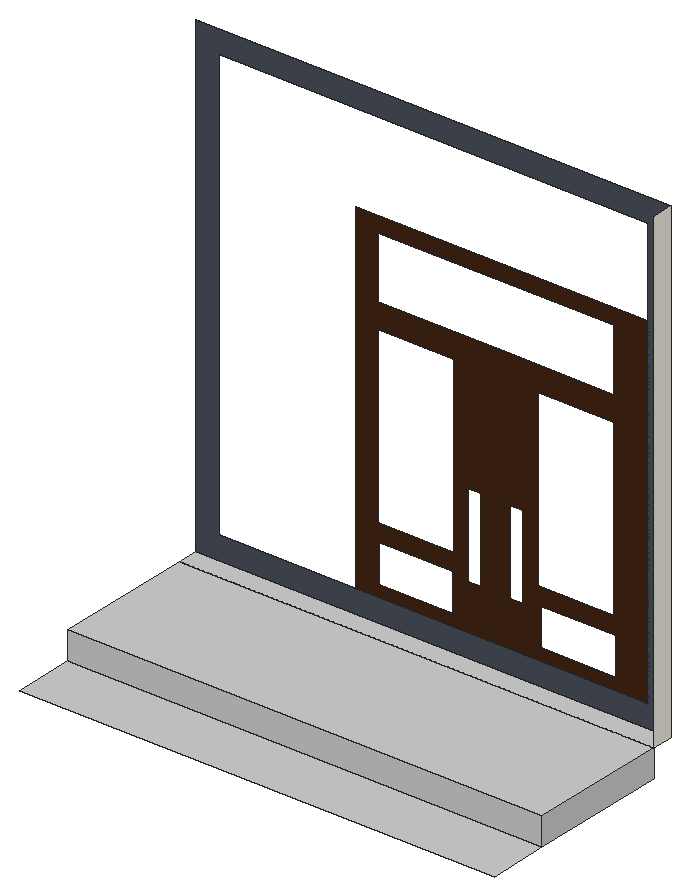
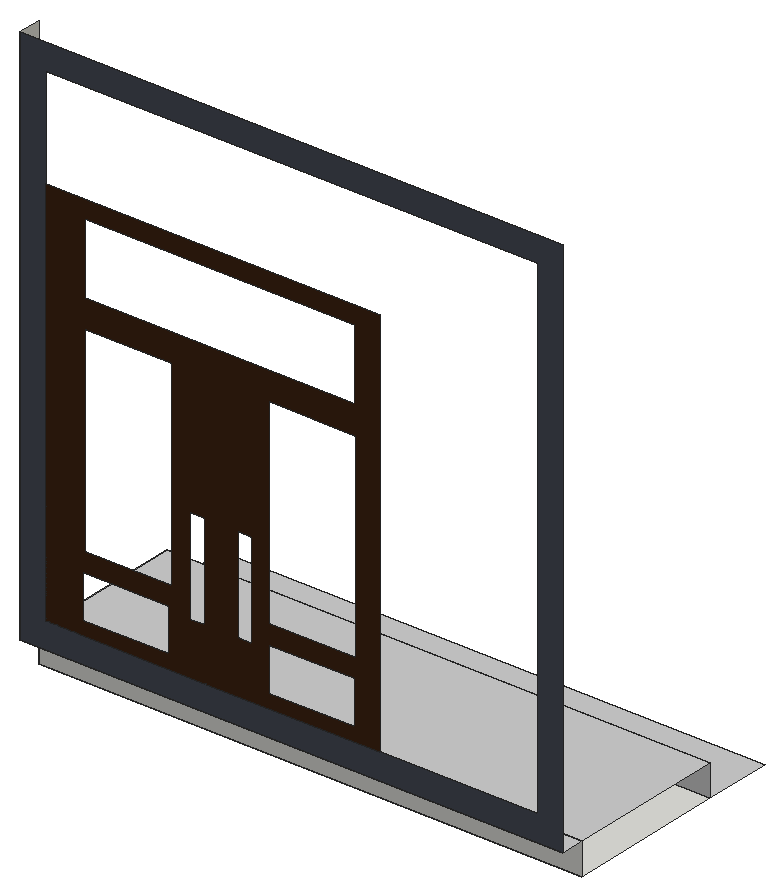
# SketchUp Ruby script. Lengths in inches.
U = 1.inch
M = Sketchup.active_model
def pt(a) = Geom::Point3d.new(a.map { |v| v * U })
def face(e, loops, mat)
  f = e.add_face(loops[0].map { |a| pt(a) })
  loops[1..].each { |l| e.add_face(l.map { |a| pt(a) }).erase! }
  f.material = f.back_material = mat if mat
  f
end
# faces: each face lists its corners as indices into pts; further lists are holes
def faces(e, pts, list, mat = nil) = list.each { |f| face(e, (f[0].is_a?(Array) ? f : [f]).map { |l| l.map { |i| pts[i] } }, mat) }
# xy, xz, yz: faces in a plane at the given z, y or x. An outline is a flat list of corners, or four numbers for a rectangle; further outlines are holes
def ring(l) = l.size == 4 ? [[l[0], l[1]], [l[2], l[1]], [l[2], l[3]], [l[0], l[3]]] : l.each_slice(2).to_a
def flat(e, list, mat, &to3) = list.each { |f| face(e, (f[0].is_a?(Array) ? f : [f]).map { |l| ring(l).map { |u, v| to3.(u, v) } }, mat) }
def xy(e, z, list, mat = nil) = flat(e, list, mat) { |x, y| [x, y, z] }
def xz(e, y, list, mat = nil) = flat(e, list, mat) { |x, z| [x, y, z] }
def yz(e, x, list, mat = nil) = flat(e, list, mat) { |y, z| [x, y, z] }
def lines(e, pts, list) = list.each { |a, b| e.add_line(pt(pts[a]), pt(pts[b])) }
# prism: a flat outline (further loops are holes) pulled along v
def prism(e, loops, v, mat = nil)
  f = face(e, loops, mat); d = Geom::Vector3d.new(v.map { |x| x * U })
  f.pushpull(f.normal.samedirection?(d) ? d.length : -d.length)
end
def box(e, o, s, mat = nil) = prism(e, [[o, [o[0] + s[0], o[1], o[2]], [o[0] + s[0], o[1] + s[1], o[2]], [o[0], o[1] + s[1], o[2]]]], [0, 0, s[2]], mat)
def at(x, y, z, deg = 0) = Geom::Transformation.translation(pt([x, y, z])) * Geom::Transformation.rotation(ORIGIN, Z_AXIS, deg.degrees)
def axes(o, x, y, z) = Geom::Transformation.new([*x, 0, *y, 0, *z, 0, *pt(o).to_a, 1])
def part(name) = M.definitions.add(name)
# library, detail: a bought-in or finely detailed component or shape, given as its bounding box
def library(name, o, s) = part(name).tap { |d| box(d.entities, o, s) }
def detail(e, o, s) = box(e.add_group.entities, o, s)
def put(e, d, t, mat = nil) = e.add_instance(d, t).tap { |i| i.material = mat if mat }
def group(e, t, mat = nil) = e.add_group.tap { |g| g.transformation = t; g.material = mat if mat }.entities
root = M.entities
M.materials.add("[Carrera Marble]").color = [207, 207, 207]
M.materials.add("[Formica Laminate Dark]").color = [74, 78, 89]
M.materials.add("[Tile Limestone Large]").color = [237, 234, 224]
M.materials.add("[Wood Veneer 01]").color = [66, 38, 20]
xy(root,70.61,[[111.93,162.11,355.29,233.86]])
xy(root,70.61,[[111.93,131.48,355.29,162.11]],"[Carrera Marble]")
xy(root,84.87,[[111.93,162.11,355.29,233.86],[111.93,233.86,355.29,244.48]],"[Carrera Marble]")
xz(root,162.11,[[111.93,70.61,355.29,84.87]],"[Carrera Marble]")
xz(root,233.86,[[111.93,70.61,355.29,84.87]])
xz(root,244.48,[[[111.93,84.87,355.29,328.93],[123.4,96.33,343.83,317.47]]],"[Formica Laminate Dark]")
xz(root,244.48,[[[193.875,96.33,265.67,96.33,265.67,232.3,205.03,232.3,205.03,264.07,326.31,264.07,326.31,232.3,265.67,232.3,265.67,96.33,343.83,96.33,343.83,272.12,193.875,272.12],[204.93,130.46,243.93,219.72],[287.31,130.46,326.31,219.72],[205.34,102.49,243.66,121.99],[288.66,102.49,326.97,121.99],[251.23,119.67,257.85,162.8],[272.6,119.67,279.23,162.8]]],"[Wood Veneer 01]")
yz(root,355.29,[[162.11,70.61,233.86,84.87]],"[Carrera Marble]")
yz(root,355.29,[[233.86,84.87,244.48,328.93]],"[Tile Limestone Large]")
